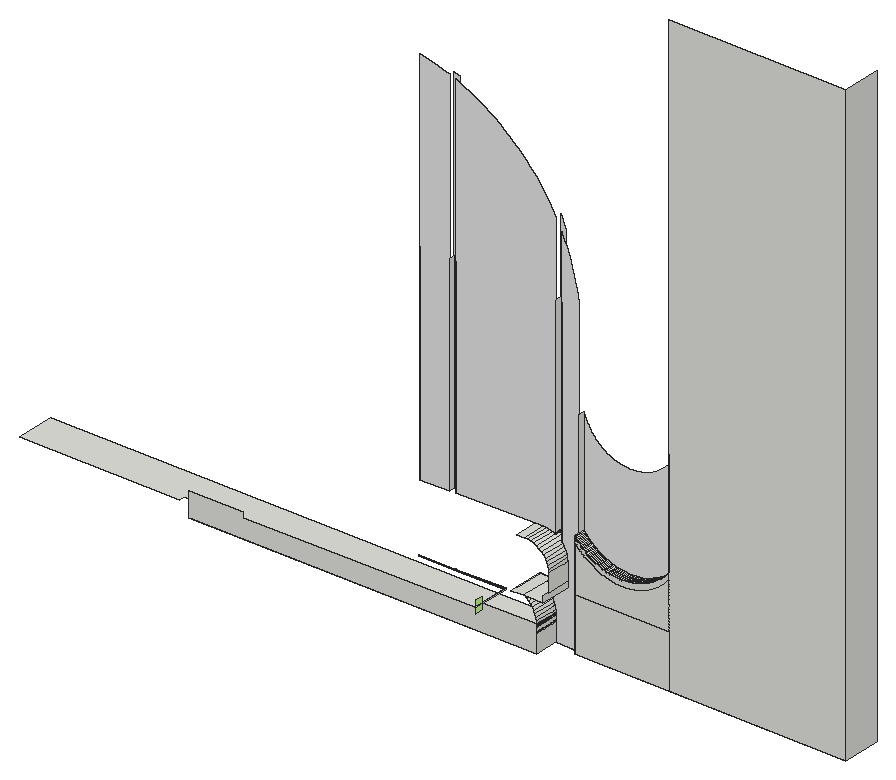
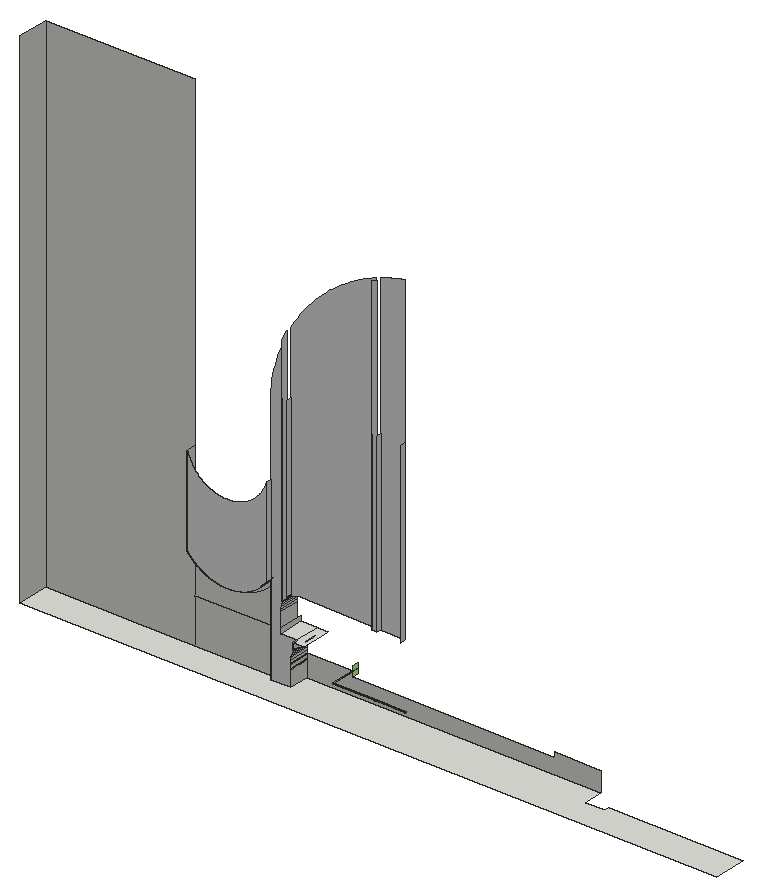
# SketchUp Ruby script. Lengths in inches.
U = 1.inch
M = Sketchup.active_model
def pt(a) = Geom::Point3d.new(a.map { |v| v * U })
def face(e, loops, mat)
  f = e.add_face(loops[0].map { |a| pt(a) })
  loops[1..].each { |l| e.add_face(l.map { |a| pt(a) }).erase! }
  f.material = f.back_material = mat if mat
  f
end
# faces: each face lists its corners as indices into pts; further lists are holes
def faces(e, pts, list, mat = nil) = list.each { |f| face(e, (f[0].is_a?(Array) ? f : [f]).map { |l| l.map { |i| pts[i] } }, mat) }
# xy, xz, yz: faces in a plane at the given z, y or x. An outline is a flat list of corners, or four numbers for a rectangle; further outlines are holes
def ring(l) = l.size == 4 ? [[l[0], l[1]], [l[2], l[1]], [l[2], l[3]], [l[0], l[3]]] : l.each_slice(2).to_a
def flat(e, list, mat, &to3) = list.each { |f| face(e, (f[0].is_a?(Array) ? f : [f]).map { |l| ring(l).map { |u, v| to3.(u, v) } }, mat) }
def xy(e, z, list, mat = nil) = flat(e, list, mat) { |x, y| [x, y, z] }
def xz(e, y, list, mat = nil) = flat(e, list, mat) { |x, z| [x, y, z] }
def yz(e, x, list, mat = nil) = flat(e, list, mat) { |y, z| [x, y, z] }
def lines(e, pts, list) = list.each { |a, b| e.add_line(pt(pts[a]), pt(pts[b])) }
# prism: a flat outline (further loops are holes) pulled along v
def prism(e, loops, v, mat = nil)
  f = face(e, loops, mat); d = Geom::Vector3d.new(v.map { |x| x * U })
  f.pushpull(f.normal.samedirection?(d) ? d.length : -d.length)
end
def box(e, o, s, mat = nil) = prism(e, [[o, [o[0] + s[0], o[1], o[2]], [o[0] + s[0], o[1] + s[1], o[2]], [o[0], o[1] + s[1], o[2]]]], [0, 0, s[2]], mat)
def at(x, y, z, deg = 0) = Geom::Transformation.translation(pt([x, y, z])) * Geom::Transformation.rotation(ORIGIN, Z_AXIS, deg.degrees)
def axes(o, x, y, z) = Geom::Transformation.new([*x, 0, *y, 0, *z, 0, *pt(o).to_a, 1])
def part(name) = M.definitions.add(name)
# library, detail: a bought-in or finely detailed component or shape, given as its bounding box
def library(name, o, s) = part(name).tap { |d| box(d.entities, o, s) }
def detail(e, o, s) = box(e.add_group.entities, o, s)
def put(e, d, t, mat = nil) = e.add_instance(d, t).tap { |i| i.material = mat if mat }
def group(e, t, mat = nil) = e.add_group.tap { |g| g.transformation = t; g.material = mat if mat }.entities
root = M.entities
M.materials.add("[Aluminum]").color = [229, 229, 229]
M.materials.add("[Color F02]").color = [204, 255, 153]
xy(root,0,[[31,1.25,31,5.25,27,5.25,27,4.25,0,4.25,0,10.75,140,10.75,140,4.25,94,4.25,94,5.25,90,5.25,90,1.25]])
xy(root,14.063,[[101.907,4.25,102.093,6.25]])
xz(root,1.25,[[31,0,90,0,90,4.47,80.688,4.396,80.688,3.396,40.112,3.073,40.104,3.973,40.104,4.073,31,4]])
xz(root,4.25,[[94,0,110,9],[110,0,140,102],[94,9,110,9,110,16.864,109.997,16.859,109.879,16.715,109.758,16.572,109.635,16.432,109.509,16.294,109.381,16.159,109.251,16.026,109.117,15.895,108.982,15.767,108.844,15.641,108.704,15.518,108.561,15.398,108.417,15.28,108.27,15.164,108.121,15.052,107.97,14.942,107.817,14.836,107.662,14.732,107.506,14.63,107.347,14.532,107.187,14.437,107.024,14.345,106.861,14.255,106.695,14.169,106.528,14.086,106.36,14.006,106.19,13.929,106.018,13.855,105.846,13.785,105.672,13.717,105.496,13.653,105.32,13.592,105.143,13.534,104.964,13.48,104.785,13.429,104.604,13.381,104.423,13.337,104.241,13.296,104.058,13.258,103.875,13.224,103.691,13.193,103.507,13.166,103.322,13.142,103.136,13.121,102.95,13.104,102.764,13.09,102.578,13.08,102.392,13.073,102.205,13.069,102.019,13.069,101.832,13.073,101.646,13.08,101.459,13.09,101.273,13.104,101.087,13.121,100.902,13.142,100.717,13.166,100.532,13.193,100.348,13.224,100.165,13.258,99.982,13.296,99.8,13.337,99.619,13.381,99.439,13.429,99.259,13.48,99.081,13.534,98.903,13.592,98.727,13.653,98.552,13.717,98.378,13.785,98.205,13.855,98.034,13.929,97.864,14.006,97.695,14.086,97.528,14.169,97.363,14.255,97.199,14.345,97.037,14.437,96.877,14.532,96.718,14.63,96.561,14.732,96.406,14.836,96.253,14.942,96.102,15.052,95.954,15.164,95.807,15.28,95.662,15.398,95.52,15.518,95.38,15.641,95.242,15.767,95.106,15.895,94.973,16.026,94.842,16.159,94.714,16.294,94.588,16.432,94.465,16.572,94.345,16.715,94.227,16.859,94.112,17.006,94,17.149],[102.019,13.069,102.205,13.069,102.392,13.073,102.578,13.08,102.764,13.09,102.95,13.104,103.136,13.121,103.322,13.142,103.507,13.166,103.691,13.193,103.875,13.224,104.058,13.258,104.241,13.296,104.423,13.337,104.604,13.381,104.785,13.429,104.964,13.48,105.143,13.534,105.32,13.592,105.496,13.653,105.672,13.717,105.846,13.785,106.018,13.855,106.19,13.929,106.36,14.006,106.528,14.086,106.695,14.169,106.861,14.255,107.024,14.345,107.187,14.437,107.347,14.532,107.506,14.63,107.662,14.732,107.817,14.836,107.97,14.942,108.121,15.052,108.27,15.164,108.417,15.28,108.561,15.398,108.704,15.518,108.844,15.641,108.982,15.767,109.117,15.895,109.251,16.026,109.381,16.159,109.509,16.294,109.635,16.432,109.758,16.572,109.879,16.715,109.997,16.859,110,16.864,110,18,109.885,17.853,109.767,17.709,109.646,17.566,109.523,17.426,109.398,17.288,109.269,17.153,109.139,17.019,109.006,16.889,108.87,16.761,108.732,16.635,108.592,16.512,108.45,16.391,108.305,16.273,108.158,16.158,108.009,16.046,107.858,15.936,107.705,15.829,107.551,15.725,107.394,15.624,107.235,15.526,107.075,15.431,106.913,15.338,106.749,15.249,106.583,15.163,106.416,15.08,106.248,15,106.078,14.923,105.907,14.849,105.734,14.778,105.56,14.711,105.385,14.647,105.208,14.586,105.031,14.528,104.852,14.474,104.673,14.423,104.493,14.375,104.311,14.331,104.129,14.29,103.947,14.252,103.763,14.218,103.579,14.187,103.395,14.159,103.21,14.135,103.024,14.115,102.839,14.097,102.653,14.084,102.466,14.073,102.28,14.066,102.093,14.063,101.907,14.063,101.72,14.066,101.534,14.073,101.347,14.084,101.161,14.097,100.976,14.115,100.79,14.135,100.605,14.159,100.421,14.187,100.237,14.218,100.053,14.252,99.871,14.29,99.689,14.331,99.507,14.375,99.327,14.423,99.148,14.474,98.969,14.528,98.792,14.586,98.615,14.647,98.44,14.711,98.266,14.778,98.093,14.849,97.922,14.923,97.752,15,97.584,15.08,97.417,15.163,97.251,15.249,97.087,15.338,96.925,15.431,96.765,15.526,96.606,15.624,96.449,15.725,96.295,15.829,96.142,15.936,95.991,16.046,95.842,16.158,95.695,16.273,95.55,16.391,95.408,16.512,95.268,16.635,95.13,16.761,94.994,16.889,94.861,17.019,94.731,17.153,94.602,17.288,94.477,17.426,94.354,17.566,94.233,17.709,94.115,17.853,94,18,94,17.149,94.112,17.006,94.227,16.859,94.345,16.715,94.465,16.572,94.588,16.432,94.714,16.294,94.842,16.159,94.973,16.026,95.106,15.895,95.242,15.767,95.38,15.641,95.52,15.518,95.662,15.398,95.807,15.28,95.954,15.164,96.102,15.052,96.253,14.942,96.406,14.836,96.561,14.732,96.718,14.63,96.877,14.532,97.037,14.437,97.199,14.345,97.363,14.255,97.528,14.169,97.695,14.086,97.864,14.006,98.034,13.929,98.205,13.855,98.378,13.785,98.552,13.717,98.727,13.653,98.903,13.592,99.081,13.534,99.259,13.48,99.439,13.429,99.619,13.381,99.8,13.337,99.982,13.296,100.165,13.258,100.348,13.224,100.532,13.193,100.717,13.166,100.902,13.142,101.087,13.121,101.273,13.104,101.459,13.09,101.646,13.08,101.832,13.073]])
xz(root,5.25,[[90,0,94,0,94,52,93.876,52.987,93.723,53.969,93.541,54.947,93.331,55.919,93.091,56.885,92.824,57.842,92.528,58.792,92.205,59.732,91.853,60.663,91.475,61.582,91.069,62.491,91,62.634,91,15.581,91.171,15.389,91.462,14.957,91.695,14.492,91.863,14,91.966,13.489,92,12.97,92,8.97,88.696,8.921,88.715,7.645,89.043,7.266,89.328,6.853,89.566,6.412,89.754,5.948,89.889,5.469,89.89,5.465,89.972,4.971,90,4.47],[90,16.4,90,64.59,89.695,65.138,89.185,65.992,88.65,66.83,88.091,67.653,87.508,68.458,86.902,69.246,86.272,70.016,85.62,70.767,84.946,71.499,84.251,72.21,83.535,72.9,82.799,73.569,82.044,74.216,81.269,74.84,80.477,75.441,79.668,76.019,78.841,76.572,77.999,77.101,77.141,77.605,76.27,78.083,75.384,78.536,74.485,78.962,73.574,79.361,73,79.593,73,16.687,86.574,16.889,88.001,16.91,88.52,16.884,89.032,16.789,89.527,16.628,89.996,16.402],[67,16.597,72,16.672,72,79.974,71.719,80.078,70.777,80.395,69.825,80.684,68.865,80.945,67.898,81.178,67,81.366]],"[Aluminum]")
xz(root,6.25,[[66,4.179,72,4.227,72,4.327,66,4.279],[72,4.227,80.688,4.296,80.688,4.396,72,4.327],[66,4.279,72,4.327,72,4.427,66,4.379],[72,4.327,80.688,4.396,80.6875,4.496,72,4.427],[88.715,7.645,88.696,8.921,86.574,8.889,87.052,8.738,87.51,8.535,87.944,8.283,88.347,7.985],
  [91,15.581,91,62.634,90.637,63.386,90.179,64.269,90,64.59,90,16.4,90.431,16.117,90.825,15.777],[72,16.672,73,16.687,73,79.593,72.652,79.733,72,79.974]])
xz(root,6.25,[[101.907,14.063,102.093,14.063,102.28,14.066,102.466,14.073,102.653,14.084,102.839,14.097,103.024,14.115,103.21,14.135,103.395,14.159,103.579,14.187,103.763,14.218,103.947,14.252,104.129,14.29,104.311,14.331,104.493,14.375,104.673,14.423,104.852,14.474,105.031,14.528,105.208,14.586,105.385,14.647,105.56,14.711,105.734,14.778,105.907,14.849,106.078,14.923,106.248,15,106.416,15.08,106.583,15.163,106.749,15.249,106.913,15.338,107.075,15.431,107.235,15.526,107.394,15.624,107.551,15.725,107.705,15.829,107.858,15.936,108.009,16.046,108.158,16.158,108.305,16.273,108.45,16.391,108.592,16.512,108.732,16.635,108.87,16.761,109.006,16.889,109.139,17.019,109.269,17.153,109.398,17.288,109.523,17.426,109.646,17.566,109.767,17.709,109.885,17.853,110,18,110,36,109.937,35.793,109.868,35.587,109.794,35.384,109.715,35.182,109.63,34.983,109.54,34.785,109.446,34.591,109.346,34.398,109.241,34.209,109.131,34.022,109.017,33.838,108.898,33.657,108.774,33.479,108.645,33.305,108.512,33.134,108.375,32.966,108.233,32.802,108.087,32.642,107.937,32.486,107.783,32.333,107.625,32.185,107.463,32.041,107.298,31.901,107.129,31.765,106.957,31.634,106.781,31.508,106.602,31.386,106.419,31.268,106.234,31.156,106.046,31.048,105.856,30.946,105.662,30.848,105.466,30.755,105.268,30.668,105.068,30.585,104.865,30.508,104.661,30.436,104.455,30.37,104.247,30.309,104.037,30.253,103.827,30.203,103.615,30.158,103.402,30.119,103.1875,30.085,102.973,30.057,102.757,30.034,102.541,30.018,102.325,30.006,102.108,30.001,101.892,30.001,101.675,30.006,101.459,30.018,101.243,30.034,101.027,30.057,100.8125,30.085,100.598,30.119,100.385,30.158,100.173,30.203,99.963,30.253,99.753,30.309,99.545,30.37,99.339,30.436,99.135,30.508,98.932,30.585,98.732,30.668,98.534,30.755,98.338,30.848,98.144,30.946,97.954,31.048,97.766,31.156,97.581,31.268,97.398,31.386,97.219,31.508,97.043,31.634,96.871,31.765,96.702,31.901,96.537,32.041,96.375,32.185,96.217,32.333,96.063,32.486,95.913,32.642,95.767,32.802,95.625,32.966,95.488,33.134,95.355,33.305,95.226,33.479,95.102,33.657,94.983,33.838,94.869,34.022,94.759,34.209,94.654,34.398,94.554,34.591,94.46,34.785,94.37,34.983,94.285,35.182,94.206,35.384,94.132,35.587,94.063,35.793,94,36,94,18,94.115,17.853,94.233,17.709,94.354,17.566,94.477,17.426,94.602,17.288,94.731,17.153,94.861,17.019,94.994,16.889,95.13,16.761,95.268,16.635,95.408,16.512,95.55,16.391,95.695,16.273,95.842,16.158,95.991,16.046,96.142,15.936,96.295,15.829,96.449,15.725,96.606,15.624,96.765,15.526,96.925,15.431,97.087,15.338,97.251,15.249,97.417,15.163,97.584,15.08,97.752,15,97.922,14.923,98.093,14.849,98.266,14.778,98.44,14.711,98.615,14.647,98.792,14.586,98.969,14.528,99.148,14.474,99.327,14.423,99.507,14.375,99.689,14.331,99.871,14.29,100.053,14.252,100.237,14.218,100.421,14.187,100.605,14.159,100.79,14.135,100.976,14.115,101.161,14.097,101.347,14.084,101.534,14.073,101.72,14.066]],"[Aluminum]")
yz(root,67,[[5.25,16.597,6.25,52]])
yz(root,72,[[5.25,16.672,6.25,52]])
yz(root,73,[[5.25,16.687,6.25,52]])
yz(root,80.688,[[1.25,4.296,6.25,4.396]])
yz(root,80.688,[[0,3.396,1.25,4.296]],"[Color F02]")
yz(root,90,[[1.25,0,5.25,3.088],[1.25,3.088,5.25,3.183],[1.25,3.183,5.25,3.231],[1.25,3.231,5.25,3.279],[1.25,3.279,5.25,3.327],
  [1.25,3.327,5.25,3.988],[1.25,3.988,5.25,4.04],[1.25,4.04,5.25,4.083],[1.25,4.083,5.25,4.088],[1.25,4.088,5.25,4.131],
  [1.25,4.131,5.25,4.179],[1.25,4.179,5.25,4.183],[1.25,4.183,5.25,4.1875],[1.25,4.1875,5.25,4.227],[1.25,4.227,5.25,4.231],
  [1.25,4.231,5.25,4.279],[1.25,4.279,5.25,4.283],[1.25,4.283,5.25,4.327],[1.25,4.327,5.25,4.331],[1.25,4.331,5.25,4.379],
  [1.25,4.379,5.25,4.427],[1.25,4.427,5.25,4.47],[5.25,16.4,6.25,16.403],[5.25,16.403,6.25,16.493],[5.25,16.493,6.25,16.582],
  [5.25,16.582,6.25,16.672],[5.25,16.672,6.25,52]])
yz(root,91,[[5.25,15.581,6.25,15.583],[5.25,15.583,6.25,16.672],[5.25,16.672,6.25,52]])
yz(root,92,[[0.125,8.97,5.25,9.97],[1.25,9.97,5.25,12.97]])
yz(root,94,[[4.25,0,5.25,9],[4.25,9,5.25,17.149],[4.25,17.149,5.25,18],[5.25,18,6.25,36]])
yz(root,110,[[4.25,18,6.25,36]])
yz(root,140,[[4.25,0,10.75,102]])
p = [[80.6875,6.25,4.496],[80.688,6.25,4.396],[80.688,1.25,4.396],[80.6875,1.25,4.496],[80.688,0,5.396],[80.6875,0,4.496],
  [80.688,1.25,5.396],[90,5.25,4.47],[89.972,5.25,4.971],[89.972,1.25,4.971],[90,1.25,4.47],[89.89,5.25,5.465],
  [89.89,1.25,5.465],[89.889,5.25,5.469],[89.754,5.25,5.948],[89.754,1.25,5.948],[89.889,1.25,5.469],[89.566,5.25,6.412],
  [89.566,1.25,6.412],[89.328,5.25,6.853],[89.328,1.25,6.853],[89.043,5.25,7.266],[89.043,1.25,7.266],[88.715,5.25,7.645],
  [88.715,1.25,7.645],[88.715,6.25,7.645],[88.347,6.25,7.985],[88.347,1.25,7.985],[88.696,6.25,8.921],[88.696,5.25,8.921],
  [87.944,6.25,8.283],[87.944,1.25,8.283],[87.51,6.25,8.535],[87.51,1.25,8.535],[87.052,6.25,8.738],[87.052,1.25,8.738],
  [86.574,6.25,8.889],[86.574,1.25,8.889],[88.696,0.125,8.921],[86.574,0.125,8.889],[92,5.25,8.97],[92,0.125,8.97],
  [92,5.25,12.97],[91.966,5.25,13.489],[91.966,1.25,13.489],[92,1.25,12.97],[91.863,5.25,14],[91.863,1.25,14],
  [91.695,5.25,14.492],[91.695,1.25,14.492],[100.79,6.25,14.135],[100.605,6.25,14.159],[100.605,4.25,14.159],[100.79,4.25,14.135],
  [100.976,6.25,14.115],[100.976,4.25,14.115],[101.161,6.25,14.097],[101.161,4.25,14.097],[101.347,6.25,14.084],[101.347,4.25,14.084],
  [101.534,6.25,14.073],[101.534,4.25,14.073],[101.72,6.25,14.066],[101.72,4.25,14.066],[101.907,6.25,14.063],[101.907,4.25,14.063],
  [102.28,6.25,14.066],[102.093,6.25,14.063],[102.093,4.25,14.063],[102.28,4.25,14.066],[102.466,6.25,14.073],[102.466,4.25,14.073],
  [102.653,6.25,14.084],[102.653,4.25,14.084],[102.839,6.25,14.097],[102.839,4.25,14.097],[103.024,6.25,14.115],[103.024,4.25,14.115],
  [103.21,6.25,14.135],[103.21,4.25,14.135],[103.395,6.25,14.159],[103.395,4.25,14.159],[100.237,6.25,14.218],[100.053,6.25,14.252],
  [100.053,4.25,14.252],[100.237,4.25,14.218],[100.421,6.25,14.187],[100.421,4.25,14.187],[103.579,6.25,14.187],[103.579,4.25,14.187],
  [103.763,6.25,14.218],[103.763,4.25,14.218],[103.947,6.25,14.252],[103.947,4.25,14.252],[99.689,6.25,14.331],[99.507,6.25,14.375],
  [99.507,4.25,14.375],[99.689,4.25,14.331],[99.871,6.25,14.29],[99.871,4.25,14.29],[104.129,6.25,14.29],[104.129,4.25,14.29],
  [104.311,6.25,14.331],[104.311,4.25,14.331],[104.493,6.25,14.375],[104.493,4.25,14.375],[99.327,6.25,14.423],[99.148,6.25,14.474],
  [99.148,4.25,14.474],[99.327,4.25,14.423],[104.673,6.25,14.423],[104.673,4.25,14.423],[104.852,6.25,14.474],[104.852,4.25,14.474],
  [91.462,5.25,14.957],[91.462,1.25,14.957],[98.969,6.25,14.528],[98.792,6.25,14.586],[98.792,4.25,14.586],[98.969,4.25,14.528],
  [105.031,6.25,14.528],[105.031,4.25,14.528],[105.208,6.25,14.586],[105.208,4.25,14.586],[98.615,6.25,14.647],[98.44,6.25,14.711],
  [98.44,4.25,14.711],[98.615,4.25,14.647],[105.385,6.25,14.647],[105.385,4.25,14.647],[105.56,6.25,14.711],[105.56,4.25,14.711],
  [98.266,6.25,14.778],[98.266,4.25,14.778],[105.734,6.25,14.778],[105.734,4.25,14.778],[98.093,6.25,14.849],[97.922,6.25,14.923],
  [97.922,4.25,14.923],[98.093,4.25,14.849],[105.907,6.25,14.849],[105.907,4.25,14.849],[106.078,6.25,14.923],[106.078,4.25,14.923],
  [97.752,6.25,15],[97.752,4.25,15],[106.248,6.25,15],[106.248,4.25,15],[91.171,5.25,15.389],[91.171,1.25,15.389],
  [97.584,6.25,15.08],[97.584,4.25,15.08],[106.416,6.25,15.08],[106.416,4.25,15.08],[97.417,6.25,15.163],[97.417,4.25,15.163],
  [106.583,6.25,15.163],[106.583,4.25,15.163],[97.251,6.25,15.249],[97.087,6.25,15.338],[97.087,4.25,15.338],[97.251,4.25,15.249],
  [106.749,6.25,15.249],[106.749,4.25,15.249],[106.913,6.25,15.338],[106.913,4.25,15.338],[96.925,6.25,15.431],[96.925,4.25,15.431],
  [107.075,6.25,15.431],[107.075,4.25,15.431],[91,5.25,15.581],[91,6.25,15.581],[90.825,6.25,15.777],[90.825,1.25,15.777],
  [91,1.25,15.581],[96.765,6.25,15.526],[96.765,4.25,15.526],[107.235,6.25,15.526],[107.235,4.25,15.526],[96.606,6.25,15.624],
  [96.606,4.25,15.624],[107.394,6.25,15.624],[107.394,4.25,15.624],[96.449,6.25,15.725],[96.449,4.25,15.725],[107.551,6.25,15.725],
  [107.551,4.25,15.725],[96.295,6.25,15.829],[96.295,4.25,15.829],[107.705,6.25,15.829],[107.705,4.25,15.829],[90.431,6.25,16.117],
  [90.431,1.25,16.117],[96.142,6.25,15.936],[96.142,4.25,15.936],[107.858,6.25,15.936],[107.858,4.25,15.936],[95.991,6.25,16.046],
  [95.991,4.25,16.046],[108.009,6.25,16.046],[108.009,4.25,16.046],[95.842,6.25,16.158],[95.842,4.25,16.158],[108.158,6.25,16.158],
  [108.158,4.25,16.158],[90,6.25,16.4],[90,5.25,16.4],[89.996,5.25,16.402],[89.996,1.25,16.402],[90,1.25,16.4],
  [95.695,6.25,16.273],[95.695,4.25,16.273],[108.305,6.25,16.273],[108.305,4.25,16.273],[95.55,6.25,16.391],[95.55,4.25,16.391],
  [108.45,6.25,16.391],[108.45,4.25,16.391],[89.527,5.25,16.628],[89.527,1.25,16.628],[95.408,6.25,16.512],[95.408,4.25,16.512],
  [108.592,6.25,16.512],[108.592,4.25,16.512],[95.268,6.25,16.635],[95.268,4.25,16.635],[108.732,6.25,16.635],[108.732,4.25,16.635],
  [89.032,5.25,16.789],[89.032,1.25,16.789],[95.13,6.25,16.761],[95.13,4.25,16.761],[108.87,6.25,16.761],[108.87,4.25,16.761],
  [88.52,5.25,16.884],[88.52,1.25,16.884],[94.994,6.25,16.889],[94.994,4.25,16.889],[109.006,6.25,16.889],[109.006,4.25,16.889],
  [88.001,5.25,16.91],[86.574,5.25,16.889],[86.574,1.25,16.889],[88.001,1.25,16.91],[94.861,6.25,17.019],[94.861,4.25,17.019],
  [109.139,6.25,17.019],[109.139,4.25,17.019],[94.731,6.25,17.153],[94.731,4.25,17.153],[109.269,6.25,17.153],[109.269,4.25,17.153],
  [94.602,6.25,17.288],[94.602,4.25,17.288],[109.398,6.25,17.288],[109.398,4.25,17.288],[94.477,6.25,17.426],[94.477,4.25,17.426],
  [109.523,6.25,17.426],[109.523,4.25,17.426],[94.354,6.25,17.566],[94.354,4.25,17.566],[109.646,6.25,17.566],[109.646,4.25,17.566],
  [94.233,6.25,17.709],[94.233,4.25,17.709],[109.767,6.25,17.709],[109.767,4.25,17.709],[94.115,6.25,17.853],[94.115,4.25,17.853],
  [109.885,6.25,17.853],[109.885,4.25,17.853],[94,6.25,18],[94,5.25,18],[94,4.25,18],[110,6.25,18],
  [110,4.25,18],[72,6.25,3.988],[72,6.25,3.327],[72,6.25,4.1875],[72,6.25,4.183],[72,6.25,5.088],
  [72,6.25,4.427],[72,6.25,4.088],[72,6.25,4.083],[72,6.25,4.131],[72,6.25,3.231],[72,6.25,3.183],
  [72,6.25,4.179],[72,6.25,4.04],[72,6.25,3.088],[72,6.25,5.183],[72,6.25,5.279],[72,6.25,5.231],
  [72,6.25,3.279],[72,6.25,5.327],[72,6.25,4.227],[67,6.25,16.597],[67,6.25,16.582],[73,6.25,16.687],
  [73,6.25,16.672]]
faces(root,p,[[0,1,2,3],[7,8,9,10],[8,11,12,9],[13,14,15,16],[11,13,16,12],[14,17,18,15],[17,19,20,18],[19,21,22,20],
  [21,23,24,22],[25,26,27,24,23],[28,25,23,29],[26,30,31,27],[30,32,33,31],[32,34,35,33],[34,36,37,35],[36,28,29,38,39,37],
  [29,40,41,38],[42,43,44,45],[43,46,47,44],[46,48,49,47],[50,51,52,53],[54,50,53,55],[56,54,55,57],[58,56,57,59],
  [60,58,59,61],[62,60,61,63],[64,62,63,65],[66,67,68,69],[70,66,69,71],[72,70,71,73],[74,72,73,75],[76,74,75,77],
  [78,76,77,79],[80,78,79,81],[82,83,84,85],[86,82,85,87],[51,86,87,52],[88,80,81,89],[90,88,89,91],[92,90,91,93],
  [94,95,96,97],[98,94,97,99],[83,98,99,84],[100,92,93,101],[102,100,101,103],[104,102,103,105],[106,107,108,109],[95,106,109,96],
  [110,104,105,111],[112,110,111,113],[48,114,115,49],[116,117,118,119],[107,116,119,108],[120,112,113,121],[122,120,121,123],[124,125,126,127],
  [117,124,127,118],[128,122,123,129],[130,128,129,131],[125,132,133,126],[134,130,131,135],[136,137,138,139],[132,136,139,133],[140,134,135,141],
  [142,140,141,143],[137,144,145,138],[146,142,143,147],[114,148,149,115],[144,150,151,145],[152,146,147,153],[150,154,155,151],[156,152,153,157],
  [158,159,160,161],[154,158,161,155],[162,156,157,163],[164,162,163,165],[159,166,167,160],[168,164,165,169],[148,170,171,172,173,174,149],[166,175,176,167],
  [177,168,169,178],[175,179,180,176],[181,177,178,182],[179,183,184,180],[185,181,182,186],[183,187,188,184],[189,185,186,190],[172,191,192,173],
  [187,193,194,188],[195,189,190,196],[193,197,198,194],[199,195,196,200],[197,201,202,198],[203,199,200,204],[205,206,207,208,209,192,191],[201,210,211,202],
  [212,203,204,213],[210,214,215,211],[216,212,213,217],[207,218,219,208],[214,220,221,215],[222,216,217,223],[220,224,225,221],[226,222,223,227],
  [218,228,229,219],[224,230,231,225],[232,226,227,233],[228,234,235,229],[230,236,237,231],[238,232,233,239],[240,241,242,243],[234,240,243,235],
  [236,244,245,237],[246,238,239,247],[244,248,249,245],[250,246,247,251],[248,252,253,249],[254,250,251,255],[252,256,257,253],[258,254,255,259],
  [256,260,261,257],[262,258,259,263],[260,264,265,261],[266,262,263,267],[264,268,269,265],[270,266,267,271],[268,272,273,274,269],[275,270,271,276]])
faces(root,p,[[4,5,3,6]],"[Color F02]")
lines(root,p,[[277,278],[279,280],[281,282],[283,284],[285,283],[286,287],[280,288],[284,289],[287,290],[291,281],[289,277],[292,293],
  [288,285],[294,286],[293,291],[295,292],[278,294],[296,279],[297,298],[299,300]])
